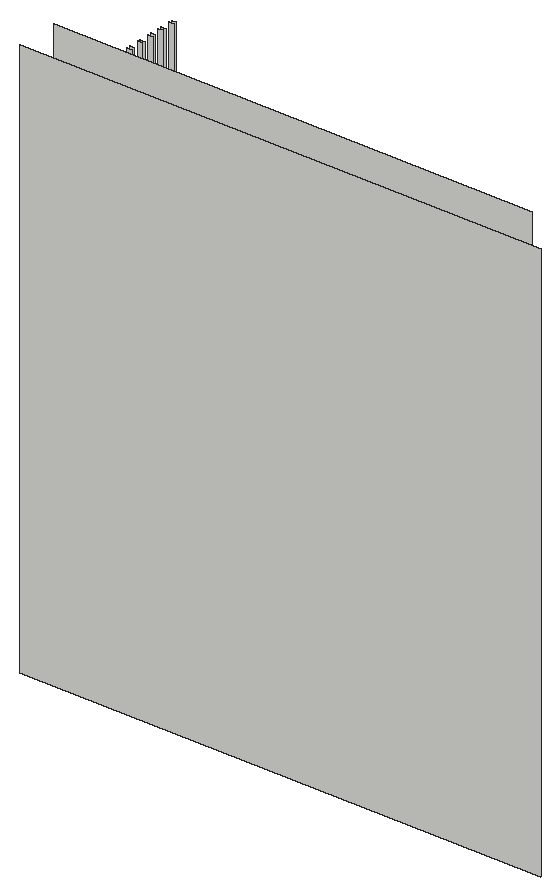
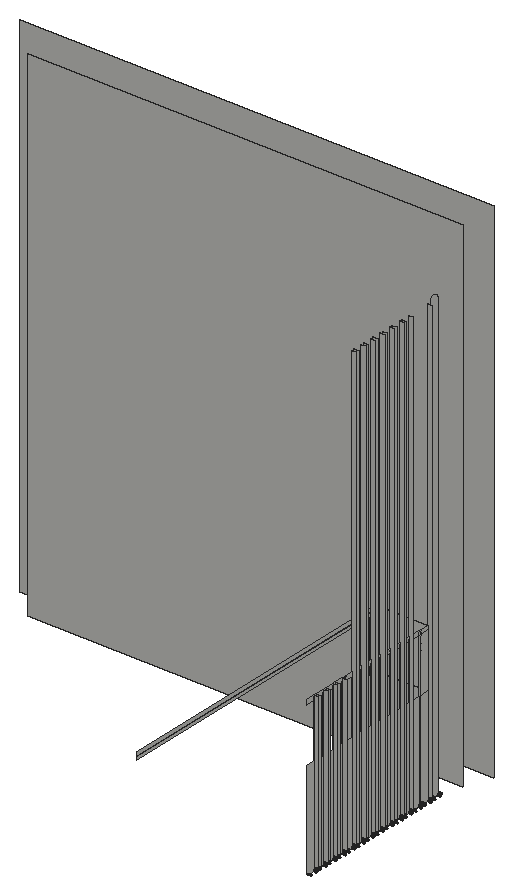
# SketchUp Ruby script. Lengths in inches.
U = 1.inch
M = Sketchup.active_model
def pt(a) = Geom::Point3d.new(a.map { |v| v * U })
def face(e, loops, mat)
  f = e.add_face(loops[0].map { |a| pt(a) })
  loops[1..].each { |l| e.add_face(l.map { |a| pt(a) }).erase! }
  f.material = f.back_material = mat if mat
  f
end
# faces: each face lists its corners as indices into pts; further lists are holes
def faces(e, pts, list, mat = nil) = list.each { |f| face(e, (f[0].is_a?(Array) ? f : [f]).map { |l| l.map { |i| pts[i] } }, mat) }
# xy, xz, yz: faces in a plane at the given z, y or x. An outline is a flat list of corners, or four numbers for a rectangle; further outlines are holes
def ring(l) = l.size == 4 ? [[l[0], l[1]], [l[2], l[1]], [l[2], l[3]], [l[0], l[3]]] : l.each_slice(2).to_a
def flat(e, list, mat, &to3) = list.each { |f| face(e, (f[0].is_a?(Array) ? f : [f]).map { |l| ring(l).map { |u, v| to3.(u, v) } }, mat) }
def xy(e, z, list, mat = nil) = flat(e, list, mat) { |x, y| [x, y, z] }
def xz(e, y, list, mat = nil) = flat(e, list, mat) { |x, z| [x, y, z] }
def yz(e, x, list, mat = nil) = flat(e, list, mat) { |y, z| [x, y, z] }
def lines(e, pts, list) = list.each { |a, b| e.add_line(pt(pts[a]), pt(pts[b])) }
# prism: a flat outline (further loops are holes) pulled along v
def prism(e, loops, v, mat = nil)
  f = face(e, loops, mat); d = Geom::Vector3d.new(v.map { |x| x * U })
  f.pushpull(f.normal.samedirection?(d) ? d.length : -d.length)
end
def box(e, o, s, mat = nil) = prism(e, [[o, [o[0] + s[0], o[1], o[2]], [o[0] + s[0], o[1] + s[1], o[2]], [o[0], o[1] + s[1], o[2]]]], [0, 0, s[2]], mat)
def at(x, y, z, deg = 0) = Geom::Transformation.translation(pt([x, y, z])) * Geom::Transformation.rotation(ORIGIN, Z_AXIS, deg.degrees)
def axes(o, x, y, z) = Geom::Transformation.new([*x, 0, *y, 0, *z, 0, *pt(o).to_a, 1])
def part(name) = M.definitions.add(name)
# library, detail: a bought-in or finely detailed component or shape, given as its bounding box
def library(name, o, s) = part(name).tap { |d| box(d.entities, o, s) }
def detail(e, o, s) = box(e.add_group.entities, o, s)
def put(e, d, t, mat = nil) = e.add_instance(d, t).tap { |i| i.material = mat if mat }
def group(e, t, mat = nil) = e.add_group.tap { |g| g.transformation = t; g.material = mat if mat }.entities
root = M.entities
xz(root,0,[[9,0,120,120]])
xz(root,9,[[9,2,111,120]])
xz(root,15.23,[[9,3.36,10,3.52]])
xz(root,17.3125,[[9,3.36,10,3.52]])
xz(root,18.02,[[9,3.36,10,3.52],[9,3.52,10,106.96],[10,25.62,22.25,39.47]])
xz(root,19.31,[[22.05,25.62,22.25,38.47]])
xz(root,19.91,[[22.05,25.62,22.25,37.86]])
xz(root,20.1,[[9,3.36,10,3.52]])
xz(root,20.81,[[9,3.36,10,3.52]])
xz(root,22.89,[[9,3.36,10,3.52]])
xz(root,23.59,[[9,3.36,10,3.52],[9,3.52,10,106.96]])
xz(root,25.67,[[9,3.29,10,3.36],[9,3.36,10,3.52],[9,3.52,10,106.96]])
xz(root,26.38,[[9,3.36,10,3.52],[9,3.52,10,106.96]])
xz(root,28.46,[[9,3.29,10,3.36],[9,3.36,10,3.52],[9,3.52,10,106.96]])
xz(root,29.17,[[9,3.36,10,3.52],[9,3.52,10,106.96]])
xz(root,31.25,[[9,3.36,10,3.52],[9,3.52,10,106.96]])
xz(root,31.96,[[9,3.29,10,3.36],[9,3.36,10,3.52],[9,3.52,10,106.96]])
xz(root,34.04,[[9,3.36,10,3.52],[9,3.52,10,106.96]])
xz(root,34.74,[[9,3.36,10,3.52],[9,3.52,10,106.96]])
xz(root,36.82,[[9,3.29,10,3.36],[9,3.36,10,3.52],[9,3.52,10,106.96]])
xz(root,37.53,[[9,3.36,10,3.52],[9,3.52,10,106.96]])
xz(root,39.61,[[9,3.29,10,3.36],[9,3.36,10,3.52],[9,3.52,10,106.96]])
xz(root,40.32,[[9,3.36,10,3.52],[9,3.52,10,106.96]])
xz(root,42.4,[[9,3.36,10,3.52]])
xz(root,43.11,[[9,3.29,10,3.36],[9,3.36,10,3.52],[9,3.52,10,39.47]])
xz(root,45.1875,[[9,3.36,10,3.52],[9,3.52,10,39.47]])
xz(root,45.89,[[9,3.36,10,3.52],[9,3.52,10,39.47]])
xz(root,47.97,[[9,3.29,10,3.36],[9,3.36,10,3.52],[9,3.52,10,39.47]])
xz(root,48.68,[[9,3.36,10,3.52],[9,3.52,10,39.47]])
xz(root,50.76,[[9,3.29,10,3.36],[9,3.36,10,3.52],[9,3.52,10,39.47]])
xz(root,51.47,[[9,3.36,10,3.52],[9,3.52,10,39.47]])
yz(root,10,[[16.16,2.4,16.39,2.4,16.44,2.41,16.5,2.42,16.55,2.44,16.61,2.45,16.66,2.47,16.72,2.5,16.77,2.52,16.87,2.58,16.91,2.62,16.96,2.65,17.08,2.77,17.23,3.02,17.25,3.07,17.27,3.125,17.28,3.18,17.3,3.24,17.31,3.29,17.3125,3.36,17.3125,107.02,17.31,107.07,17.29,107.18,17.28,107.23,17.2,107.43,17.14,107.53,17.11,107.57,17.08,107.62,17.05,107.66,17.01,107.7,16.97,107.73,16.93,107.77,16.88,107.8,16.84,107.83,16.74,107.89,16.7,107.91,16.64,107.93,16.54,107.97,16.49,107.98,16.43,107.99,16.38,108,16.16,108,16.06,107.98,16,107.97,15.8,107.89,15.7,107.83,15.62,107.77,15.58,107.73,15.54,107.7,15.46,107.62,15.43,107.57,15.4,107.53,15.34,107.43,15.28,107.28,15.27,107.23,15.25,107.18,15.24,107.125,15.24,107.07,15.23,107.02,15.23,3.36,15.24,3.29,15.25,3.24,15.26,3.18,15.3,3.07,15.34,2.97,15.43,2.82,15.47,2.77,15.59,2.65,15.63,2.62,15.68,2.58,15.78,2.52,15.83,2.5,15.88,2.47,15.93,2.45,15.99,2.44,16.04,2.42],[18.94,2.4,19.17,2.4,19.29,2.42,19.34,2.44,19.4,2.45,19.45,2.47,19.5,2.5,19.55,2.52,19.65,2.58,19.7,2.62,19.74,2.65,19.79,2.69,19.83,2.73,19.86,2.77,19.9,2.82,19.99,2.97,20.01,3.02,20.04,3.07,20.05,3.125,20.07,3.18,20.08,3.24,20.09,3.29,20.1,3.36,20.1,25.62,18.02,25.62,18.02,3.36,18.03,3.29,18.04,3.24,18.05,3.18,18.0625,3.125,18.08,3.07,18.1,3.02,18.16,2.92,18.1875,2.87,18.22,2.82,18.26,2.77,18.29,2.73,18.33,2.69,18.375,2.65,18.42,2.62,18.47,2.58,18.51,2.55,18.5625,2.52,18.61,2.5,18.67,2.47,18.72,2.45,18.78,2.44,18.83,2.42,18.89,2.41],[21.73,2.4,21.96,2.4,22.02,2.41,22.07,2.42,22.13,2.44,22.18,2.45,22.24,2.47,22.29,2.5,22.34,2.52,22.44,2.58,22.49,2.62,22.53,2.65,22.65,2.77,22.6875,2.82,22.72,2.87,22.78,2.97,22.82,3.07,22.86,3.18,22.87,3.24,22.88,3.29,22.89,3.36,22.89,25.62,20.81,25.62,20.81,3.36,20.8125,3.29,20.82,3.24,20.84,3.18,20.85,3.125,20.87,3.07,20.89,3.02,20.92,2.97,20.94,2.92,20.97,2.87,21.01,2.82,21.04,2.77,21.16,2.65,21.21,2.62,21.25,2.58,21.35,2.52,21.4,2.5,21.46,2.47,21.51,2.45,21.5625,2.44,21.62,2.42,21.68,2.41],[24.52,2.4,24.75,2.4,24.81,2.41,24.86,2.42,24.92,2.44,24.97,2.45,25.03,2.47,25.08,2.5,25.13,2.52,25.23,2.58,25.27,2.62,25.32,2.65,25.4,2.73,25.4375,2.77,25.47,2.82,25.51,2.87,25.54,2.92,25.5625,2.97,25.59,3.02,25.61,3.07,25.65,3.18,25.66,3.24,25.67,3.29,25.67,25.62,23.59,25.62,23.59,3.36,23.6,3.29,23.61,3.24,23.625,3.18,23.64,3.125,23.66,3.07,23.7,2.97,23.79,2.82,23.83,2.77,23.95,2.65,23.99,2.62,24.04,2.58,24.14,2.52,24.19,2.5,24.24,2.47,24.3,2.45,24.35,2.44,24.41,2.42,24.46,2.41],[27.31,2.4,27.54,2.4,27.59,2.41,27.65,2.42,27.7,2.44,27.76,2.45,27.8125,2.47,27.87,2.5,27.92,2.52,28.02,2.58,28.0625,2.62,28.11,2.65,28.15,2.69,28.1875,2.73,28.23,2.77,28.35,2.97,28.4,3.07,28.42,3.125,28.43,3.18,28.45,3.24,28.46,3.29,28.46,25.62,26.38,25.62,26.38,3.36,26.39,3.29,26.4,3.24,26.41,3.18,26.45,3.07,26.49,2.97,26.58,2.82,26.62,2.77,26.74,2.65,26.78,2.62,26.83,2.58,26.875,2.55,26.93,2.52,26.98,2.5,27.03,2.47,27.08,2.45,27.14,2.44,27.19,2.42],
  [30.09,2.4,30.32,2.4,30.38,2.41,30.4375,2.42,30.49,2.44,30.55,2.45,30.6,2.47,30.65,2.5,30.7,2.52,30.8,2.58,30.85,2.62,30.89,2.65,30.94,2.69,30.98,2.73,31.01,2.77,31.05,2.82,31.14,2.97,31.16,3.02,31.1875,3.07,31.2,3.125,31.22,3.18,31.23,3.24,31.24,3.29,31.25,3.36,31.25,25.62,29.17,25.62,29.17,3.36,29.18,3.29,29.1875,3.24,29.2,3.18,29.21,3.125,29.23,3.07,29.25,3.02,29.37,2.82,29.41,2.77,29.44,2.73,29.48,2.69,29.53,2.65,29.57,2.62,29.62,2.58,29.66,2.55,29.71,2.52,29.76,2.5,29.82,2.47,29.87,2.45,29.93,2.44,29.98,2.42,30.04,2.41],[32.88,2.4,33.11,2.4,33.17,2.41,33.22,2.42,33.28,2.44,33.33,2.45,33.39,2.47,33.44,2.5,33.49,2.52,33.59,2.58,33.64,2.62,33.68,2.65,33.8,2.77,33.84,2.82,33.93,2.97,33.97,3.07,34.01,3.18,34.02,3.24,34.03,3.29,34.04,3.36,34.04,25.62,31.96,25.62,31.96,3.29,31.97,3.24,31.99,3.18,32,3.125,32.02,3.07,32.04,3.02,32.07,2.97,32.09,2.92,32.16,2.82,32.19,2.77,32.27,2.69,32.3125,2.65,32.36,2.62,32.4,2.58,32.5,2.52,32.55,2.5,32.61,2.47,32.66,2.45,32.71,2.44,32.77,2.42,32.83,2.41],[35.67,2.4,35.9,2.4,35.96,2.41,36.01,2.42,36.07,2.44,36.12,2.45,36.18,2.47,36.23,2.5,36.28,2.52,36.38,2.58,36.42,2.62,36.47,2.65,36.59,2.77,36.66,2.87,36.6875,2.92,36.71,2.97,36.74,3.02,36.76,3.07,36.8,3.18,36.81,3.24,36.82,3.29,36.82,25.62,34.74,25.62,34.74,3.36,34.75,3.29,34.76,3.24,34.77,3.18,34.81,3.07,34.85,2.97,34.94,2.82,34.98,2.77,35.1,2.65,35.14,2.62,35.19,2.58,35.29,2.52,35.34,2.5,35.39,2.47,35.45,2.45,35.5,2.44,35.56,2.42,35.61,2.41],[38.46,2.4,38.6875,2.4,38.74,2.41,38.8,2.42,38.85,2.44,38.91,2.45,38.96,2.47,39.02,2.5,39.07,2.52,39.17,2.58,39.21,2.62,39.26,2.65,39.34,2.73,39.375,2.77,39.41,2.82,39.53,3.02,39.55,3.07,39.57,3.125,39.58,3.18,39.6,3.24,39.61,3.29,39.61,25.62,37.53,25.62,37.53,3.36,37.54,3.29,37.55,3.24,37.5625,3.18,37.58,3.125,37.6,3.07,37.64,2.97,37.73,2.82,37.77,2.77,37.89,2.65,37.93,2.62,37.98,2.58,38.08,2.52,38.13,2.5,38.18,2.47,38.23,2.45,38.29,2.44,38.34,2.42],[41.24,2.4,41.47,2.4,41.59,2.42,41.64,2.44,41.7,2.45,41.75,2.47,41.8,2.5,41.85,2.52,41.95,2.58,42,2.62,42.04,2.65,42.09,2.69,42.16,2.77,42.2,2.82,42.29,2.97,42.3125,3.02,42.34,3.07,42.35,3.125,42.37,3.18,42.38,3.24,42.39,3.29,42.4,3.36,42.4,25.62,40.32,25.62,40.32,3.36,40.33,3.29,40.34,3.24,40.35,3.18,40.36,3.125,40.38,3.07,40.4,3.02,40.52,2.82,40.56,2.77,40.59,2.73,40.63,2.69,40.68,2.65,40.72,2.62,40.77,2.58,40.8125,2.55,40.86,2.52,40.91,2.5,40.97,2.47,41.02,2.45,41.08,2.44,41.13,2.42,41.1875,2.41],
  [44.03,2.4,44.26,2.4,44.32,2.41,44.375,2.42,44.43,2.44,44.48,2.45,44.54,2.47,44.59,2.5,44.64,2.52,44.74,2.58,44.79,2.62,44.83,2.65,44.95,2.77,44.99,2.82,45.08,2.97,45.1,3.02,45.125,3.07,45.14,3.125,45.16,3.18,45.17,3.24,45.18,3.29,45.1875,3.36,45.1875,25.62,43.11,25.62,43.11,3.29,43.125,3.24,43.14,3.18,43.15,3.125,43.17,3.07,43.19,3.02,43.22,2.97,43.24,2.92,43.27,2.87,43.31,2.82,43.34,2.77,43.46,2.65,43.51,2.62,43.55,2.58,43.65,2.52,43.7,2.5,43.76,2.47,43.81,2.45,43.86,2.44,43.92,2.42,43.98,2.41],[46.82,2.4,47.05,2.4,47.11,2.41,47.16,2.42,47.22,2.44,47.27,2.45,47.33,2.47,47.38,2.5,47.43,2.52,47.53,2.58,47.57,2.62,47.62,2.65,47.74,2.77,47.77,2.82,47.81,2.87,47.84,2.92,47.86,2.97,47.89,3.02,47.91,3.07,47.95,3.18,47.96,3.24,47.97,3.29,47.97,25.62,45.89,25.62,45.89,3.36,45.9,3.29,45.91,3.24,45.92,3.18,45.9375,3.125,45.96,3.07,46,2.97,46.03,2.92,46.0625,2.87,46.09,2.82,46.13,2.77,46.25,2.65,46.29,2.62,46.34,2.58,46.39,2.55,46.4375,2.52,46.49,2.5,46.54,2.47,46.6,2.45,46.65,2.44,46.71,2.42,46.76,2.41],[49.61,2.4,49.84,2.4,49.89,2.41,49.95,2.42,50,2.44,50.06,2.45,50.11,2.47,50.17,2.5,50.22,2.52,50.32,2.58,50.36,2.62,50.41,2.65,50.53,2.77,50.5625,2.82,50.59,2.87,50.625,2.92,50.65,2.97,50.68,3.02,50.7,3.07,50.72,3.125,50.73,3.18,50.75,3.24,50.76,3.29,50.76,25.62,48.68,25.62,48.68,3.36,48.6875,3.29,48.7,3.24,48.71,3.18,48.75,3.07,48.79,2.97,48.88,2.82,48.92,2.77,49.04,2.65,49.08,2.62,49.13,2.58,49.23,2.52,49.28,2.5,49.33,2.47,49.38,2.45,49.4375,2.44,49.49,2.42],[52.39,2.4,52.625,2.4,52.68,2.41,52.74,2.42,52.79,2.44,52.85,2.45,52.9,2.47,52.95,2.5,53,2.52,53.1,2.58,53.15,2.62,53.19,2.65,53.24,2.69,53.28,2.73,53.3125,2.77,53.35,2.82,53.41,2.92,53.4375,2.97,53.46,3.02,53.49,3.07,53.5,3.125,53.52,3.18,53.53,3.24,53.54,3.29,53.55,3.36,53.55,25.62,51.47,25.62,51.47,3.36,51.48,3.29,51.49,3.24,51.5,3.18,51.51,3.125,51.53,3.07,51.55,3.02,51.67,2.82,51.71,2.77,51.74,2.73,51.78,2.69,51.83,2.65,51.87,2.62,51.92,2.58,51.96,2.55,52.01,2.52,52.06,2.5,52.12,2.47,52.17,2.45,52.23,2.44,52.28,2.42,52.34,2.41],[18.02,25.62,20.1,38.47],
  [20.1,25.62,20.81,38.47],[22.89,25.62,23.59,38.47],[25.67,25.62,26.38,38.47],[28.46,25.62,29.17,38.47],[31.25,25.62,31.96,38.47],
  [34.04,25.62,34.74,38.47],[36.82,25.62,37.53,38.47],[39.61,25.62,40.32,38.47],[42.4,25.62,43.11,38.47],[45.1875,25.62,45.89,38.47],
  [47.97,25.62,48.68,38.47],[50.76,25.62,51.47,38.47],[18.02,38.47,20.1,39.47],[20.1,38.47,20.81,39.47],[20.81,38.47,22.89,39.47],
  [22.89,38.47,23.59,39.47],[23.59,38.47,25.67,39.47],[25.67,38.47,26.38,39.47],[26.38,38.47,28.46,39.47],[28.46,38.47,29.17,39.47],
  [29.17,38.47,31.25,39.47],[31.25,38.47,31.96,39.47],[31.96,38.47,34.04,39.47],[34.04,38.47,34.74,39.47],[34.74,38.47,36.82,39.47],
  [36.82,38.47,37.53,39.47],[37.53,38.47,39.61,39.47],[39.61,38.47,40.32,39.47],[40.32,38.47,42.02,39.47],[42.02,38.47,42.4,39.47],
  [42.4,38.47,43.11,39.47],[43.11,38.47,45.1875,39.47],[45.1875,38.47,45.89,39.47],[45.89,38.47,47.97,39.47],[47.97,38.47,48.68,39.47],
  [48.68,38.47,50.76,39.47],[50.76,38.47,51.47,39.47],[51.47,38.47,53.55,39.47]])
yz(root,22.05,[[19.31,25.62,19.91,25.62,19.91,37.86,88.07,37.86,88.07,38.47,19.31,38.47]])
yz(root,22.25,[[18.02,25.62,19.31,25.62,19.31,38.47,88.07,38.47,88.07,39.47,18.02,39.47]])
p = [[9,15.47,2.77],[9,15.51,2.73],[10,15.51,2.73],[10,15.47,2.77],[9,15.55,2.69],[10,15.55,2.69],
  [9,17.04,2.73],[9,17.08,2.77],[10,17.08,2.77],[10,17.04,2.73],[9,18.26,2.77],[9,18.29,2.73],
  [10,18.29,2.73],[10,18.26,2.77],[9,18.33,2.69],[10,18.33,2.69],[9,19.83,2.73],[9,19.86,2.77],
  [10,19.86,2.77],[10,19.83,2.73],[9,21.04,2.77],[9,21.08,2.73],[10,21.08,2.73],[10,21.04,2.77],
  [9,21.12,2.69],[10,21.12,2.69],[9,22.61,2.73],[9,22.65,2.77],[10,22.65,2.77],[10,22.61,2.73],
  [9,23.83,2.77],[9,23.87,2.73],[10,23.87,2.73],[10,23.83,2.77],[9,23.91,2.69],[10,23.91,2.69],
  [9,25.4,2.73],[9,25.4375,2.77],[10,25.4375,2.77],[10,25.4,2.73],[9,26.62,2.77],[9,26.66,2.73],
  [10,26.66,2.73],[10,26.62,2.77],[9,26.7,2.69],[10,26.7,2.69],[9,28.1875,2.73],[9,28.23,2.77],
  [10,28.23,2.77],[10,28.1875,2.73],[9,29.41,2.77],[9,29.44,2.73],[10,29.44,2.73],[10,29.41,2.77],
  [9,29.48,2.69],[10,29.48,2.69],[9,30.98,2.73],[9,31.01,2.77],[10,31.01,2.77],[10,30.98,2.73],
  [9,32.19,2.77],[9,32.23,2.73],[10,32.23,2.73],[10,32.19,2.77],[9,32.27,2.69],[10,32.27,2.69],
  [9,33.76,2.73],[9,33.8,2.77],[10,33.8,2.77],[10,33.76,2.73],[9,34.98,2.77],[9,35.02,2.73],
  [10,35.02,2.73],[10,34.98,2.77],[9,35.06,2.69],[10,35.06,2.69],[9,36.55,2.73],[9,36.59,2.77],
  [10,36.59,2.77],[10,36.55,2.73],[9,37.77,2.77],[9,37.81,2.73],[10,37.81,2.73],[10,37.77,2.77],
  [9,37.85,2.69],[10,37.85,2.69],[9,39.34,2.73],[9,39.375,2.77],[10,39.375,2.77],[10,39.34,2.73],
  [9,40.56,2.77],[9,40.59,2.73],[10,40.59,2.73],[10,40.56,2.77],[9,40.63,2.69],[10,40.63,2.69],
  [9,42.125,2.73],[9,42.16,2.77],[10,42.16,2.77],[10,42.125,2.73],[9,43.34,2.77],[9,43.38,2.73],
  [10,43.38,2.73],[10,43.34,2.77],[9,43.42,2.69],[10,43.42,2.69],[9,44.91,2.73],[9,44.95,2.77],
  [10,44.95,2.77],[10,44.91,2.73],[9,46.13,2.77],[9,46.17,2.73],[10,46.17,2.73],[10,46.13,2.77],
  [9,46.21,2.69],[10,46.21,2.69],[9,47.7,2.73],[9,47.74,2.77],[10,47.74,2.77],[10,47.7,2.73],
  [9,48.92,2.77],[9,48.96,2.73],[10,48.96,2.73],[10,48.92,2.77],[9,49,2.69],[10,49,2.69],
  [9,50.49,2.73],[9,50.53,2.77],[10,50.53,2.77],[10,50.49,2.73],[9,51.71,2.77],[9,51.74,2.73],
  [10,51.74,2.73],[10,51.71,2.77],[9,51.78,2.69],[10,51.78,2.69],[9,53.28,2.73],[9,53.3125,2.77],
  [10,53.3125,2.77],[10,53.28,2.73],[9,15.4,2.87],[9,15.43,2.82],[10,15.43,2.82],[10,15.4,2.87],
  [9,17.11,2.82],[10,17.11,2.82],[9,17.14,2.87],[10,17.14,2.87],[9,18.1875,2.87],[9,18.22,2.82],
  [10,18.22,2.82],[10,18.1875,2.87],[9,19.9,2.82],[10,19.9,2.82],[9,19.93,2.87],[10,19.93,2.87],
  [9,20.97,2.87],[9,21.01,2.82],[10,21.01,2.82],[10,20.97,2.87],[9,22.6875,2.82],[10,22.6875,2.82],
  [9,22.72,2.87],[10,22.72,2.87],[9,23.76,2.87],[9,23.79,2.82],[10,23.79,2.82],[10,23.76,2.87],
  [9,25.47,2.82],[10,25.47,2.82],[9,25.51,2.87],[10,25.51,2.87],[9,26.55,2.87],[9,26.58,2.82],
  [10,26.58,2.82],[10,26.55,2.87],[9,28.26,2.82],[10,28.26,2.82],[9,28.29,2.87],[10,28.29,2.87],
  [9,29.34,2.87],[9,29.37,2.82],[10,29.37,2.82],[10,29.34,2.87],[9,31.05,2.82],[10,31.05,2.82],
  [9,31.08,2.87],[10,31.08,2.87],[9,32.125,2.87],[9,32.16,2.82],[10,32.16,2.82],[10,32.125,2.87],
  [9,33.84,2.82],[10,33.84,2.82],[9,33.87,2.87],[10,33.87,2.87],[9,34.91,2.87],[9,34.94,2.82],
  [10,34.94,2.82],[10,34.91,2.87],[9,36.625,2.82],[10,36.625,2.82],[9,36.66,2.87],[10,36.66,2.87],
  [9,37.7,2.87],[9,37.73,2.82],[10,37.73,2.82],[10,37.7,2.87],[9,39.41,2.82],[10,39.41,2.82],
  [9,39.44,2.87],[10,39.44,2.87],[9,40.49,2.87],[9,40.52,2.82],[10,40.52,2.82],[10,40.49,2.87],
  [9,42.2,2.82],[10,42.2,2.82],[9,42.23,2.87],[10,42.23,2.87],[9,43.27,2.87],[9,43.31,2.82],
  [10,43.31,2.82],[10,43.27,2.87],[9,44.99,2.82],[10,44.99,2.82],[9,45.02,2.87],[10,45.02,2.87],
  [9,46.0625,2.87],[9,46.09,2.82],[10,46.09,2.82],[10,46.0625,2.87],[9,47.77,2.82],[10,47.77,2.82],
  [9,47.81,2.87],[10,47.81,2.87],[9,48.85,2.87],[9,48.88,2.82],[10,48.88,2.82],[10,48.85,2.87],
  [9,50.5625,2.82],[10,50.5625,2.82],[9,50.59,2.87],[10,50.59,2.87],[9,51.64,2.87],[9,51.67,2.82],
  [10,51.67,2.82],[10,51.64,2.87],[9,53.35,2.82],[10,53.35,2.82],[9,53.38,2.87],[10,53.38,2.87],
  [9,15.34,2.97],[9,15.37,2.92],[10,15.37,2.92],[10,15.34,2.97],[9,17.17,2.92],[10,17.17,2.92],
  [9,17.2,2.97],[10,17.2,2.97],[9,18.13,2.97],[9,18.16,2.92],[10,18.16,2.92],[10,18.13,2.97],
  [9,19.96,2.92],[10,19.96,2.92],[9,19.99,2.97],[10,19.99,2.97],[9,20.92,2.97],[9,20.94,2.92],
  [10,20.94,2.92],[10,20.92,2.97],[9,22.75,2.92],[10,22.75,2.92],[9,22.78,2.97],[10,22.78,2.97],
  [9,23.7,2.97],[9,23.73,2.92],[10,23.73,2.92],[10,23.7,2.97],[9,25.54,2.92],[10,25.54,2.92],
  [9,25.5625,2.97],[10,25.5625,2.97],[9,26.49,2.97],[9,26.52,2.92],[10,26.52,2.92],[10,26.49,2.97],
  [9,28.32,2.92],[10,28.32,2.92],[9,28.35,2.97],[10,28.35,2.97],[9,29.28,2.97],[9,29.31,2.92],
  [10,29.31,2.92],[10,29.28,2.97],[9,31.11,2.92],[10,31.11,2.92],[9,31.14,2.97],[10,31.14,2.97],
  [9,32.07,2.97],[9,32.09,2.92],[10,32.09,2.92],[10,32.07,2.97],[9,33.9,2.92],[10,33.9,2.92],
  [9,33.93,2.97],[10,33.93,2.97],[9,34.85,2.97],[9,34.88,2.92],[10,34.88,2.92],[10,34.85,2.97],
  [9,36.6875,2.92],[10,36.6875,2.92],[9,36.71,2.97],[10,36.71,2.97],[9,37.64,2.97],[9,37.67,2.92],
  [10,37.67,2.92],[10,37.64,2.97],[9,39.47,2.92],[10,39.47,2.92],[9,39.5,2.97],[10,39.5,2.97],
  [9,40.43,2.97],[9,40.46,2.92],[10,40.46,2.92],[10,40.43,2.97],[9,42.26,2.92],[10,42.26,2.92],
  [9,42.29,2.97],[10,42.29,2.97],[9,43.22,2.97],[9,43.24,2.92],[10,43.24,2.92],[10,43.22,2.97],
  [9,45.05,2.92],[10,45.05,2.92],[9,45.08,2.97],[10,45.08,2.97],[9,46,2.97],[9,46.03,2.92],
  [10,46.03,2.92],[10,46,2.97],[9,47.84,2.92],[10,47.84,2.92],[9,47.86,2.97],[10,47.86,2.97],
  [9,48.79,2.97],[9,48.82,2.92],[10,48.82,2.92],[10,48.79,2.97],[9,50.625,2.92],[10,50.625,2.92],
  [9,50.65,2.97],[10,50.65,2.97],[9,51.58,2.97],[9,51.61,2.92],[10,51.61,2.92],[10,51.58,2.97],
  [9,53.41,2.92],[10,53.41,2.92],[9,53.4375,2.97],[10,53.4375,2.97],[9,15.3,3.07],[9,15.32,3.02],
  [10,15.32,3.02],[10,15.3,3.07],[9,17.23,3.02],[10,17.23,3.02],[9,17.25,3.07],[10,17.25,3.07],
  [9,18.08,3.07],[9,18.1,3.02],[10,18.1,3.02],[10,18.08,3.07],[9,20.01,3.02],[10,20.01,3.02],
  [9,20.04,3.07],[10,20.04,3.07],[9,20.87,3.07],[9,20.89,3.02],[10,20.89,3.02],[10,20.87,3.07],
  [9,22.8,3.02],[10,22.8,3.02],[9,22.82,3.07],[10,22.82,3.07],[9,23.66,3.07],[9,23.68,3.02],
  [10,23.68,3.02],[10,23.66,3.07],[9,25.59,3.02],[10,25.59,3.02],[9,25.61,3.07],[10,25.61,3.07],
  [9,26.45,3.07],[9,26.47,3.02],[10,26.47,3.02],[10,26.45,3.07],[9,28.375,3.02],[10,28.375,3.02],
  [9,28.4,3.07],[10,28.4,3.07],[9,29.23,3.07],[9,29.25,3.02],[10,29.25,3.02],[10,29.23,3.07],
  [9,31.16,3.02],[10,31.16,3.02],[9,31.1875,3.07],[10,31.1875,3.07],[9,32.02,3.07],[9,32.04,3.02],
  [10,32.04,3.02],[10,32.02,3.07],[9,33.95,3.02],[10,33.95,3.02],[9,33.97,3.07],[10,33.97,3.07],
  [9,34.81,3.07],[9,34.83,3.02],[10,34.83,3.02],[10,34.81,3.07],[9,36.74,3.02],[10,36.74,3.02],
  [9,36.76,3.07],[10,36.76,3.07],[9,37.6,3.07],[9,37.62,3.02],[10,37.62,3.02],[10,37.6,3.07],
  [9,39.53,3.02],[10,39.53,3.02],[9,39.55,3.07],[10,39.55,3.07],[9,40.38,3.07],[9,40.4,3.02],
  [10,40.4,3.02],[10,40.38,3.07],[9,42.3125,3.02],[10,42.3125,3.02],[9,42.34,3.07],[10,42.34,3.07],
  [9,43.17,3.07],[9,43.19,3.02],[10,43.19,3.02],[10,43.17,3.07],[9,45.1,3.02],[10,45.1,3.02],
  [9,45.125,3.07],[10,45.125,3.07],[9,45.96,3.07],[9,45.98,3.02],[10,45.98,3.02],[10,45.96,3.07],
  [9,47.89,3.02],[10,47.89,3.02],[9,47.91,3.07],[10,47.91,3.07],[9,48.75,3.07],[9,48.77,3.02],
  [10,48.77,3.02],[10,48.75,3.07],[9,50.68,3.02],[10,50.68,3.02],[9,50.7,3.07],[10,50.7,3.07],
  [9,51.53,3.07],[9,51.55,3.02],[10,51.55,3.02],[10,51.53,3.07],[9,53.46,3.02],[10,53.46,3.02],
  [9,15.26,3.18],[9,15.28,3.125],[10,15.28,3.125],[10,15.26,3.18],[9,17.27,3.125],[10,17.27,3.125],
  [9,17.28,3.18],[10,17.28,3.18],[9,18.05,3.18],[9,18.0625,3.125],[10,18.0625,3.125],[10,18.05,3.18],
  [9,20.05,3.125],[10,20.05,3.125],[9,20.07,3.18],[10,20.07,3.18],[9,20.84,3.18],[9,20.85,3.125],
  [10,20.85,3.125],[10,20.84,3.18],[9,22.84,3.125],[10,22.84,3.125],[9,22.86,3.18],[10,22.86,3.18],
  [9,23.625,3.18],[9,23.64,3.125],[10,23.64,3.125],[10,23.625,3.18],[9,25.63,3.125],[10,25.63,3.125],
  [9,25.65,3.18],[10,25.65,3.18],[9,26.41,3.18],[9,26.43,3.125],[10,26.43,3.125],[10,26.41,3.18],
  [9,28.42,3.125],[10,28.42,3.125],[9,28.43,3.18],[10,28.43,3.18],[9,29.2,3.18],[9,29.21,3.125],
  [10,29.21,3.125],[10,29.2,3.18],[9,31.2,3.125],[10,31.2,3.125],[9,31.22,3.18],[10,31.22,3.18],
  [9,31.99,3.18],[9,32,3.125],[10,32,3.125],[10,31.99,3.18],[9,33.99,3.125],[10,33.99,3.125],
  [9,34.01,3.18],[10,34.01,3.18],[9,34.77,3.18],[9,34.79,3.125],[10,34.79,3.125],[10,34.77,3.18],
  [9,36.78,3.125],[10,36.78,3.125],[9,36.8,3.18],[10,36.8,3.18],[9,37.5625,3.18],[9,37.58,3.125],
  [10,37.58,3.125],[10,37.5625,3.18],[9,39.57,3.125],[10,39.57,3.125],[9,39.58,3.18],[10,39.58,3.18],
  [9,40.35,3.18],[9,40.36,3.125],[10,40.36,3.125],[10,40.35,3.18],[9,42.35,3.125],[10,42.35,3.125],
  [9,42.37,3.18],[10,42.37,3.18],[9,43.14,3.18],[9,43.15,3.125],[10,43.15,3.125],[10,43.14,3.18],
  [9,45.14,3.125],[10,45.14,3.125],[9,45.16,3.18],[10,45.16,3.18],[9,45.92,3.18],[9,45.9375,3.125],
  [10,45.9375,3.125],[10,45.92,3.18],[9,47.93,3.125],[10,47.93,3.125],[9,47.95,3.18],[10,47.95,3.18],
  [9,48.71,3.18],[9,48.73,3.125],[10,48.73,3.125],[10,48.71,3.18],[9,50.72,3.125],[10,50.72,3.125],
  [9,50.73,3.18],[10,50.73,3.18],[9,51.5,3.18],[9,51.51,3.125],[10,51.51,3.125],[10,51.5,3.18],
  [9,15.24,3.29],[9,15.25,3.24],[10,15.25,3.24],[10,15.24,3.29],[9,17.3,3.24],[10,17.3,3.24],
  [9,17.31,3.29],[10,17.31,3.29],[9,18.03,3.29],[9,18.04,3.24],[10,18.04,3.24],[10,18.03,3.29],
  [9,20.08,3.24],[10,20.08,3.24],[9,20.09,3.29],[10,20.09,3.29],[9,20.8125,3.29],[9,20.82,3.24],
  [10,20.82,3.24],[10,20.8125,3.29],[9,22.87,3.24],[10,22.87,3.24],[9,22.88,3.29],[10,22.88,3.29],
  [9,23.6,3.29],[9,23.61,3.24],[10,23.61,3.24],[10,23.6,3.29],[9,25.66,3.24],[10,25.66,3.24],
  [9,25.67,3.29],[10,25.67,3.29],[9,26.39,3.29],[9,26.4,3.24],[10,26.4,3.24],[10,26.39,3.29],
  [9,28.45,3.24],[10,28.45,3.24],[9,28.46,3.29],[10,28.46,3.29],[9,29.18,3.29],[9,29.1875,3.24],
  [10,29.1875,3.24],[10,29.18,3.29],[9,31.23,3.24],[10,31.23,3.24],[9,31.24,3.29],[10,31.24,3.29],
  [9,31.96,3.29],[9,31.97,3.24],[10,31.97,3.24],[10,31.96,3.29],[9,34.02,3.24],[10,34.02,3.24],
  [9,34.03,3.29],[10,34.03,3.29],[9,34.75,3.29],[9,34.76,3.24],[10,34.76,3.24],[10,34.75,3.29],
  [9,36.81,3.24],[10,36.81,3.24],[9,36.82,3.29],[10,36.82,3.29],[9,37.54,3.29],[9,37.55,3.24],
  [10,37.55,3.24],[10,37.54,3.29],[9,39.6,3.24],[10,39.6,3.24],[9,39.61,3.29],[10,39.61,3.29],
  [9,40.33,3.29],[9,40.34,3.24],[10,40.34,3.24],[10,40.33,3.29],[9,42.38,3.24],[10,42.38,3.24],
  [9,42.39,3.29],[10,42.39,3.29],[9,43.11,3.29],[9,43.125,3.24],[10,43.125,3.24],[10,43.11,3.29],
  [9,45.17,3.24],[10,45.17,3.24],[9,45.18,3.29],[10,45.18,3.29],[9,45.9,3.29],[9,45.91,3.24],
  [10,45.91,3.24],[10,45.9,3.29],[9,47.96,3.24],[10,47.96,3.24],[9,47.97,3.29],[10,47.97,3.29],
  [9,48.6875,3.29],[9,48.7,3.24],[10,48.7,3.24],[10,48.6875,3.29],[9,50.75,3.24],[10,50.75,3.24],
  [9,50.76,3.29],[10,50.76,3.29],[9,51.48,3.29],[9,51.49,3.24],[10,51.49,3.24],[10,51.48,3.29],
  [9,15.23,3.36],[10,15.23,3.36],[9,17.3125,3.36],[10,17.3125,3.36],[9,18.02,3.36],[10,18.02,3.36],
  [9,20.1,3.36],[10,20.1,3.36],[9,20.81,3.36],[10,20.81,3.36],[9,22.89,3.36],[10,22.89,3.36],
  [9,23.59,3.36],[10,23.59,3.36],[9,26.38,3.36],[10,26.38,3.36],[9,29.17,3.36],[10,29.17,3.36],
  [9,31.25,3.36],[10,31.25,3.36],[9,34.04,3.36],[10,34.04,3.36],[9,34.74,3.36],[10,34.74,3.36],
  [9,37.53,3.36],[10,37.53,3.36],[9,40.32,3.36],[10,40.32,3.36],[9,42.4,3.36],[10,42.4,3.36],
  [9,45.1875,3.36],[10,45.1875,3.36],[9,45.89,3.36],[10,45.89,3.36],[9,48.68,3.36],[10,48.68,3.36],
  [9,51.47,3.36],[10,51.47,3.36]]
faces(root,p,[[0,1,2,3],[1,4,5,2],[6,7,8,9],[10,11,12,13],[11,14,15,12],[16,17,18,19],[20,21,22,23],[21,24,25,22],
  [26,27,28,29],[30,31,32,33],[31,34,35,32],[36,37,38,39],[40,41,42,43],[41,44,45,42],[46,47,48,49],[50,51,52,53],
  [51,54,55,52],[56,57,58,59],[60,61,62,63],[61,64,65,62],[66,67,68,69],[70,71,72,73],[71,74,75,72],[76,77,78,79],
  [80,81,82,83],[81,84,85,82],[86,87,88,89],[90,91,92,93],[91,94,95,92],[96,97,98,99],[100,101,102,103],[101,104,105,102],
  [106,107,108,109],[110,111,112,113],[111,114,115,112],[116,117,118,119],[120,121,122,123],[121,124,125,122],[126,127,128,129],[130,131,132,133],
  [131,134,135,132],[136,137,138,139],[140,141,142,143],[141,0,3,142],[7,144,145,8],[144,146,147,145],[148,149,150,151],[149,10,13,150],
  [17,152,153,18],[152,154,155,153],[156,157,158,159],[157,20,23,158],[27,160,161,28],[160,162,163,161],[164,165,166,167],[165,30,33,166],
  [37,168,169,38],[168,170,171,169],[172,173,174,175],[173,40,43,174],[47,176,177,48],[176,178,179,177],[180,181,182,183],[181,50,53,182],
  [57,184,185,58],[184,186,187,185],[188,189,190,191],[189,60,63,190],[67,192,193,68],[192,194,195,193],[196,197,198,199],[197,70,73,198],
  [77,200,201,78],[200,202,203,201],[204,205,206,207],[205,80,83,206],[87,208,209,88],[208,210,211,209],[212,213,214,215],[213,90,93,214],
  [97,216,217,98],[216,218,219,217],[220,221,222,223],[221,100,103,222],[107,224,225,108],[224,226,227,225],[228,229,230,231],[229,110,113,230],
  [117,232,233,118],[232,234,235,233],[236,237,238,239],[237,120,123,238],[127,240,241,128],[240,242,243,241],[244,245,246,247],[245,130,133,246],
  [137,248,249,138],[248,250,251,249],[252,253,254,255],[253,140,143,254],[146,256,257,147],[256,258,259,257],[260,261,262,263],[261,148,151,262],
  [154,264,265,155],[264,266,267,265],[268,269,270,271],[269,156,159,270],[162,272,273,163],[272,274,275,273],[276,277,278,279],[277,164,167,278],
  [170,280,281,171],[280,282,283,281],[284,285,286,287],[285,172,175,286],[178,288,289,179],[288,290,291,289],[292,293,294,295],[293,180,183,294],
  [186,296,297,187],[296,298,299,297],[300,301,302,303],[301,188,191,302],[194,304,305,195],[304,306,307,305],[308,309,310,311],[309,196,199,310],
  [202,312,313,203],[312,314,315,313],[316,317,318,319],[317,204,207,318],[210,320,321,211],[320,322,323,321],[324,325,326,327],[325,212,215,326],
  [218,328,329,219],[328,330,331,329],[332,333,334,335],[333,220,223,334],[226,336,337,227],[336,338,339,337],[340,341,342,343],[341,228,231,342],
  [234,344,345,235],[344,346,347,345],[348,349,350,351],[349,236,239,350],[242,352,353,243],[352,354,355,353],[356,357,358,359],[357,244,247,358],
  [250,360,361,251],[360,362,363,361],[364,365,366,367],[365,252,255,366],[258,368,369,259],[368,370,371,369],[372,373,374,375],[373,260,263,374],
  [266,376,377,267],[376,378,379,377],[380,381,382,383],[381,268,271,382],[274,384,385,275],[384,386,387,385],[388,389,390,391],[389,276,279,390],
  [282,392,393,283],[392,394,395,393],[396,397,398,399],[397,284,287,398],[290,400,401,291],[400,402,403,401],[404,405,406,407],[405,292,295,406],
  [298,408,409,299],[408,410,411,409],[412,413,414,415],[413,300,303,414],[306,416,417,307],[416,418,419,417],[420,421,422,423],[421,308,311,422],
  [314,424,425,315],[424,426,427,425],[428,429,430,431],[429,316,319,430],[322,432,433,323],[432,434,435,433],[436,437,438,439],[437,324,327,438],
  [330,440,441,331],[440,442,443,441],[444,445,446,447],[445,332,335,446],[338,448,449,339],[448,450,451,449],[452,453,454,455],[453,340,343,454],
  [346,456,457,347],[456,458,459,457],[460,461,462,463],[461,348,351,462],[354,464,465,355],[464,466,467,465],[468,469,470,471],[469,356,359,470],
  [362,472,473,363],[474,475,476,477],[475,364,367,476],[370,478,479,371],[478,480,481,479],[482,483,484,485],[483,372,375,484],[378,486,487,379],
  [486,488,489,487],[490,491,492,493],[491,380,383,492],[386,494,495,387],[494,496,497,495],[498,499,500,501],[499,388,391,500],[394,502,503,395],
  [502,504,505,503],[506,507,508,509],[507,396,399,508],[402,510,511,403],[510,512,513,511],[514,515,516,517],[515,404,407,516],[410,518,519,411],
  [518,520,521,519],[522,523,524,525],[523,412,415,524],[418,526,527,419],[526,528,529,527],[530,531,532,533],[531,420,423,532],[426,534,535,427],
  [534,536,537,535],[538,539,540,541],[539,428,431,540],[434,542,543,435],[542,544,545,543],[546,547,548,549],[547,436,439,548],[442,550,551,443],
  [550,552,553,551],[554,555,556,557],[555,444,447,556],[450,558,559,451],[558,560,561,559],[562,563,564,565],[563,452,455,564],[458,566,567,459],
  [566,568,569,567],[570,571,572,573],[571,460,463,572],[466,574,575,467],[574,576,577,575],[578,579,580,581],[579,468,471,580],[582,583,584,585],
  [583,474,477,584],[480,586,587,481],[586,588,589,587],[590,591,592,593],[591,482,485,592],[488,594,595,489],[594,596,597,595],[598,599,600,601],
  [599,490,493,600],[496,602,603,497],[602,604,605,603],[606,607,608,609],[607,498,501,608],[504,610,611,505],[610,612,613,611],[614,615,616,617],
  [615,506,509,616],[512,618,619,513],[618,620,621,619],[622,623,624,625],[623,514,517,624],[520,626,627,521],[626,628,629,627],[630,631,632,633],
  [631,522,525,632],[528,634,635,529],[634,636,637,635],[638,639,640,641],[639,530,533,640],[536,642,643,537],[642,644,645,643],[646,647,648,649],
  [647,538,541,648],[544,650,651,545],[650,652,653,651],[654,655,656,657],[655,546,549,656],[552,658,659,553],[658,660,661,659],[662,663,664,665],
  [663,554,557,664],[560,666,667,561],[666,668,669,667],[670,671,672,673],[671,562,565,672],[568,674,675,569],[674,676,677,675],[678,679,680,681],
  [679,570,573,680],[576,682,683,577],[682,684,685,683],[686,687,688,689],[687,578,581,688],[690,582,585,691],[588,692,693,589],[694,590,593,695],
  [596,696,697,597],[698,598,601,699],[604,700,701,605],[702,606,609,703],[704,614,617,705],[706,622,625,707],[628,708,709,629],[636,710,711,637],
  [712,638,641,713],[714,646,649,715],[716,654,657,717],[660,718,719,661],[668,720,721,669],[722,670,673,723],[724,678,681,725],[726,686,689,727]])
